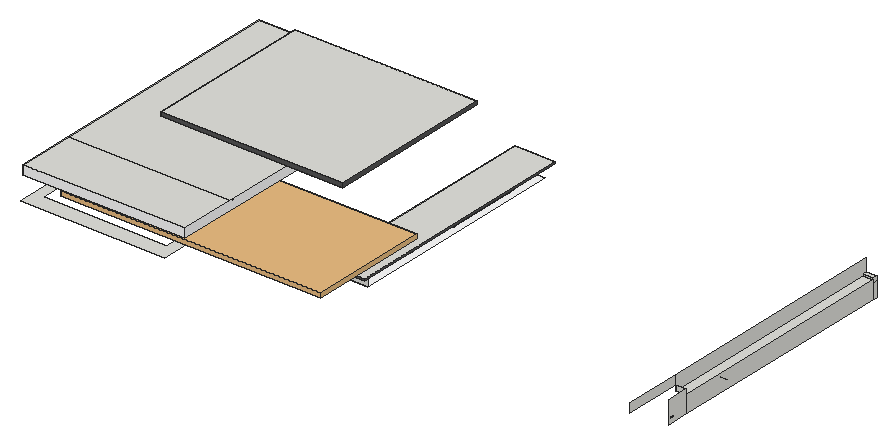
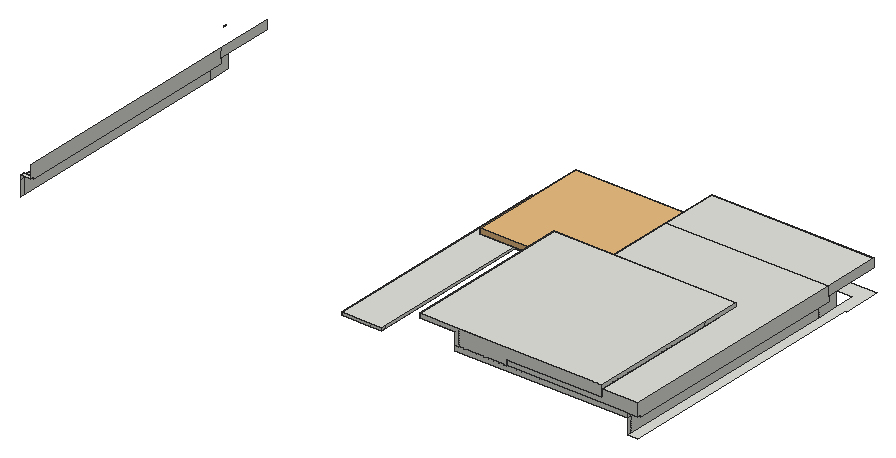
# SketchUp Ruby script. Lengths in inches.
U = 1.inch
M = Sketchup.active_model
def pt(a) = Geom::Point3d.new(a.map { |v| v * U })
def face(e, loops, mat)
  f = e.add_face(loops[0].map { |a| pt(a) })
  loops[1..].each { |l| e.add_face(l.map { |a| pt(a) }).erase! }
  f.material = f.back_material = mat if mat
  f
end
# faces: each face lists its corners as indices into pts; further lists are holes
def faces(e, pts, list, mat = nil) = list.each { |f| face(e, (f[0].is_a?(Array) ? f : [f]).map { |l| l.map { |i| pts[i] } }, mat) }
# xy, xz, yz: faces in a plane at the given z, y or x. An outline is a flat list of corners, or four numbers for a rectangle; further outlines are holes
def ring(l) = l.size == 4 ? [[l[0], l[1]], [l[2], l[1]], [l[2], l[3]], [l[0], l[3]]] : l.each_slice(2).to_a
def flat(e, list, mat, &to3) = list.each { |f| face(e, (f[0].is_a?(Array) ? f : [f]).map { |l| ring(l).map { |u, v| to3.(u, v) } }, mat) }
def xy(e, z, list, mat = nil) = flat(e, list, mat) { |x, y| [x, y, z] }
def xz(e, y, list, mat = nil) = flat(e, list, mat) { |x, z| [x, y, z] }
def yz(e, x, list, mat = nil) = flat(e, list, mat) { |y, z| [x, y, z] }
def lines(e, pts, list) = list.each { |a, b| e.add_line(pt(pts[a]), pt(pts[b])) }
# prism: a flat outline (further loops are holes) pulled along v
def prism(e, loops, v, mat = nil)
  f = face(e, loops, mat); d = Geom::Vector3d.new(v.map { |x| x * U })
  f.pushpull(f.normal.samedirection?(d) ? d.length : -d.length)
end
def box(e, o, s, mat = nil) = prism(e, [[o, [o[0] + s[0], o[1], o[2]], [o[0] + s[0], o[1] + s[1], o[2]], [o[0], o[1] + s[1], o[2]]]], [0, 0, s[2]], mat)
def at(x, y, z, deg = 0) = Geom::Transformation.translation(pt([x, y, z])) * Geom::Transformation.rotation(ORIGIN, Z_AXIS, deg.degrees)
def axes(o, x, y, z) = Geom::Transformation.new([*x, 0, *y, 0, *z, 0, *pt(o).to_a, 1])
def part(name) = M.definitions.add(name)
# library, detail: a bought-in or finely detailed component or shape, given as its bounding box
def library(name, o, s) = part(name).tap { |d| box(d.entities, o, s) }
def detail(e, o, s) = box(e.add_group.entities, o, s)
def put(e, d, t, mat = nil) = e.add_instance(d, t).tap { |i| i.material = mat if mat }
def group(e, t, mat = nil) = e.add_group.tap { |g| g.transformation = t; g.material = mat if mat }.entities
root = M.entities
M.materials.add("[Color M00]").color = [255, 255, 255]
M.materials.add("[Color M06]").color = [86, 86, 86]
c1 = library("Mesh Light\#4",[-0.5,-0.5,-0.1],[1,1,0.2])
c2 = part("Group\#24")
xy(c2.entities,0,[[203.13,95.41,201.58,95.62,200.13,96.22,198.89,97.17,197.9375,98.41,197.34,99.86,197.13,101.41,197.34,102.96,197.9375,104.41,198.89,105.65,200.13,106.61,201.58,107.21,203.13,107.41,204.6875,107.21,206.13,106.61,207.375,105.65,208.33,104.41,208.93,102.96,209.13,101.41,208.93,99.86,208.33,98.41,207.375,97.17,206.13,96.22,204.6875,95.62],[281.57,95.41,280.02,95.62,278.57,96.22,277.33,97.17,276.375,98.41,275.77,99.86,275.57,101.41,275.77,102.96,276.375,104.41,277.33,105.65,278.57,106.61,280.02,107.21,281.57,107.41,283.125,107.21,284.57,106.61,285.8125,105.65,286.77,104.41,287.37,102.96,287.57,101.41,287.37,99.86,286.77,98.41,285.8125,97.17,284.57,96.22,283.125,95.62],[350.95,95.41,349.39,95.62,347.95,96.22,346.7,97.17,345.75,98.41,345.15,99.86,344.95,101.41,345.15,102.96,345.75,104.41,346.7,105.65,347.95,106.61,349.39,107.21,350.95,107.41,352.5,107.21,353.95,106.61,355.1875,105.65,356.14,104.41,356.74,102.96,356.95,101.41,356.74,99.86,356.14,98.41,355.1875,97.17,353.95,96.22,352.5,95.62],[376,162.85,374.44,163.05,373,163.65,371.75,164.6,370.8,165.85,370.2,167.29,370,168.85,370.2,170.4,370.8,171.85,371.75,173.09,373,174.04,374.44,174.64,376,174.85,377.55,174.64,379,174.04,380.24,173.09,381.19,171.85,381.79,170.4,382,168.85,381.79,167.29,381.19,165.85,380.24,164.6,379,163.65,377.55,163.05]],"[Color M00]")
xy(c2.entities,33.4375,[[6,0,4.45,0.2,3,0.8,1.76,1.76,0.8,3,0.2,4.45,0,6,0.2,7.55,0.8,9,1.76,10.24,3,11.2,4.45,11.8,6,12,7.55,11.8,9,11.2,10.24,10.24,11.2,9,11.8,7.55,12,6,11.8,4.45,11.2,3,10.24,1.76,9,0.8,7.55,0.2],[83.125,0,81.57,0.2,80.125,0.8,78.88,1.76,77.93,3,77.33,4.45,77.125,6,77.33,7.55,77.93,9,78.88,10.24,80.125,11.2,81.57,11.8,83.125,12,84.68,11.8,86.125,11.2,87.37,10.24,88.32,9,88.92,7.55,89.125,6,88.92,4.45,88.32,3,87.37,1.76,86.125,0.8,84.68,0.2],[166.6875,0,165.13,0.2,163.6875,0.8,162.44,1.76,161.49,3,160.89,4.45,160.6875,6,160.89,7.55,161.49,9,162.44,10.24,163.6875,11.2,165.13,11.8,166.6875,12,168.24,11.8,169.6875,11.2,170.93,10.24,171.88,9,172.48,7.55,172.6875,6,172.48,4.45,171.88,3,170.93,1.76,169.6875,0.8,168.24,0.2],[166.6875,88.9375,165.13,89.14,163.6875,89.74,162.44,90.69,161.49,91.9375,160.89,93.38,160.6875,94.9375,160.89,96.49,161.49,97.9375,162.44,99.18,163.6875,100.13,165.13,100.73,166.6875,100.9375,168.24,100.73,169.6875,100.13,170.93,99.18,171.88,97.9375,172.48,96.49,172.6875,94.9375,172.48,93.38,171.88,91.9375,170.93,90.69,169.6875,89.74,168.24,89.14]],"[Color M00]")
put(c2.entities,c1,axes([191,87.42,16.72],[382.99758,0,0],[0,175.84579,0],[0,0,34.4375]))
c3 = library("Group\#23",[-0.5,-0.5,-0.1],[13,110.375,0.2])
xy(root,269.375,[[278.36,1583.41,490.8,1583.41,490.8,1676.03,484.3,1676.03,484.3,1705.53,475.29,1705.53,475.29,1606.6875,294.47,1606.6875,294.47,2020.66,279.74,2020.66,279.74,1638.35,278.36,1638.35],[484.3,1676.03,490.8,1730.6]])
xy(root,269.375,[[[490.8,1676.03,490.8,1730.6,674.49,1730.6,674.49,2001.02,715.11,2001.02,715.11,1676.03],[604.45,1698.07,606.01,1698.28,607.45,1698.875,608.7,1699.83,609.65,1701.07,610.25,1702.52,610.45,1704.07,610.25,1705.625,609.65,1707.07,608.7,1708.3125,607.45,1709.27,606.01,1709.87,604.45,1710.07,602.9,1709.87,601.45,1709.27,600.21,1708.3125,599.26,1707.07,598.66,1705.625,598.45,1704.07,598.66,1702.52,599.26,1701.07,600.21,1699.83,601.45,1698.875,602.9,1698.28],[673.83,1698.07,675.38,1698.28,676.83,1698.875,678.07,1699.83,679.02,1701.07,679.625,1702.52,679.83,1704.07,679.625,1705.625,679.02,1707.07,678.07,1708.3125,676.83,1709.27,675.38,1709.87,673.83,1710.07,672.27,1709.87,670.83,1709.27,669.59,1708.3125,668.63,1707.07,668.03,1705.625,667.83,1704.07,668.03,1702.52,668.63,1701.07,669.59,1699.83,670.83,1698.875,672.27,1698.28],[526.02,1698.07,527.57,1698.28,529.02,1698.875,530.26,1699.83,531.21,1701.07,531.8125,1702.52,532.02,1704.07,531.8125,1705.625,531.21,1707.07,530.26,1708.3125,529.02,1709.27,527.57,1709.87,526.02,1710.07,524.46,1709.87,523.02,1709.27,521.77,1708.3125,520.82,1707.07,520.22,1705.625,520.02,1704.07,520.22,1702.52,520.82,1701.07,521.77,1699.83,523.02,1698.875,524.46,1698.28],[698.88,1943.32,700.43,1943.52,701.88,1944.12,703.12,1945.08,704.08,1946.32,704.68,1947.77,704.88,1949.32,704.68,1950.87,704.08,1952.32,703.12,1953.5625,701.88,1954.51,700.43,1955.11,698.88,1955.32,697.33,1955.11,695.88,1954.51,694.64,1953.5625,693.68,1952.32,693.08,1950.87,692.88,1949.32,693.08,1947.77,693.68,1946.32,694.64,1945.08,695.88,1944.12,697.33,1943.52],[698.88,1765.51,700.43,1765.71,701.88,1766.31,703.12,1767.26,704.08,1768.51,704.68,1769.95,704.88,1771.51,704.68,1773.06,704.08,1774.51,703.12,1775.75,701.88,1776.7,700.43,1777.3,698.88,1777.51,697.33,1777.3,695.88,1776.7,694.64,1775.75,693.68,1774.51,693.08,1773.06,692.88,1771.51,693.08,1769.95,693.68,1768.51,694.64,1767.26,695.88,1766.31,697.33,1765.71],[698.88,1845.94,700.43,1846.15,701.88,1846.75,703.12,1847.7,704.08,1848.94,704.68,1850.39,704.88,1851.94,704.68,1853.5,704.08,1854.94,703.12,1856.1875,701.88,1857.14,700.43,1857.74,698.88,1857.94,697.33,1857.74,695.88,1857.14,694.64,1856.1875,693.68,1854.94,693.08,1853.5,692.88,1851.94,693.08,1850.39,693.68,1848.94,694.64,1847.7,695.88,1846.75,697.33,1846.15]]],"[Color M00]")
xy(root,279.25,[[484.3,1669.78,715.11,1676.03],[484.3,1676.03,484.3,1775.97,655.66,1775.97,655.66,2020.66,715.11,2020.66,715.11,1676.03]])
xy(root,282.6875,[[484.3,1669.78,715.11,1669.78,715.11,2020.66,655.66,2020.66,655.66,1775.97,484.3,1775.97]])
xy(root,291.125,[[304.78,1733.11,304.78,2014.29,471.68,2014.29,471.68,1853.85,462.15,1853.85,462.15,1733.11],[471.68,1853.85,542.11,2014.29]])
xy(root,294.9375,[[279.74,1669.84,294.47,2014.29],[1172.33,1669.84,1187.0625,2014.29]])
xy(root,297.875,[[279.74,2014.29,294.47,2020.66],[294.47,2014.29,471.68,2020.66],[471.68,2014.29,542.11,2020.66],[1172.33,2014.29,1187.0625,2020.66]])
xy(root,302.8125,[[[279.74,1586.53,279.74,1669.84,294.47,1669.84,294.47,1638.53,471.68,1638.53,471.68,1831.47,518.11,1831.47,518.11,1586.53],[328.88,1602.66,330.44,1602.86,331.88,1603.46,333.125,1604.42,334.08,1605.66,334.68,1607.11,334.88,1608.66,334.68,1610.21,334.08,1611.66,333.125,1612.9,331.88,1613.86,330.44,1614.46,328.88,1614.66,327.33,1614.46,325.88,1613.86,324.64,1612.9,323.6875,1611.66,323.09,1610.21,322.88,1608.66,323.09,1607.11,323.6875,1605.66,324.64,1604.42,325.88,1603.46,327.33,1602.86],[406.01,1602.66,407.56,1602.86,409.01,1603.46,410.25,1604.42,411.2,1605.66,411.8,1607.11,412.01,1608.66,411.8,1610.21,411.2,1611.66,410.25,1612.9,409.01,1613.86,407.56,1614.46,406.01,1614.66,404.45,1614.46,403.01,1613.86,401.76,1612.9,400.8125,1611.66,400.21,1610.21,400.01,1608.66,400.21,1607.11,400.8125,1605.66,401.76,1604.42,403.01,1603.46,404.45,1602.86],[489.57,1602.66,491.12,1602.86,492.57,1603.46,493.8125,1604.42,494.77,1605.66,495.37,1607.11,495.57,1608.66,495.37,1610.21,494.77,1611.66,493.8125,1612.9,492.57,1613.86,491.12,1614.46,489.57,1614.66,488.02,1614.46,486.57,1613.86,485.33,1612.9,484.375,1611.66,483.77,1610.21,483.57,1608.66,483.77,1607.11,484.375,1605.66,485.33,1604.42,486.57,1603.46,488.02,1602.86],[489.57,1691.6,491.12,1691.8,492.57,1692.4,493.8125,1693.35,494.77,1694.6,495.37,1696.04,495.57,1697.6,495.37,1699.15,494.77,1700.6,493.8125,1701.84,492.57,1702.79,491.12,1703.39,489.57,1703.6,488.02,1703.39,486.57,1702.79,485.33,1701.84,484.375,1700.6,483.77,1699.15,483.57,1697.6,483.77,1696.04,484.375,1694.6,485.33,1693.35,486.57,1692.4,488.02,1691.8]]],"[Color M00]")
xy(root,305.625,[[332.11,1831.47,471.68,2020.66]])
xy(root,316.0625,[[279.74,1586.53,518.11,1669.84],[279.74,1669.84,518.11,1669.84,518.11,1773.85,332.11,1773.85,332.11,2020.66,279.74,2020.66],[518.11,1773.85,518.11,1831.47,548.11,1831.47,548.11,2020.66,599.68,2020.66,599.68,1773.85]])
xy(root,321.8125,[[332.11,1773.85,599.68,2020.66]])
xz(root,1586.53,[[279.74,302.8125,518.11,316.0625]],"[Color M00]")
xz(root,1669.78,[[484.3,279.25,715.11,282.6875]],"[Color M06]")
xz(root,1669.84,[[279.74,294.9375,294.47,302.8125],[1172.33,294.9375,1187.0625,302.8125]])
xz(root,1676.03,[[484.3,269.375,715.11,279.25]])
xz(root,1773.85,[[332.11,316.0625,599.68,321.8125]],"[Color M06]")
xz(root,1775.97,[[484.3,279.25,655.66,282.6875]])
xz(root,1831.47,[[471.68,302.8125,518.11,305.625]])
xz(root,2014.29,[[294.47,291.125,471.68,297.875],[471.68,291.125,542.11,297.875],[279.74,294.9375,294.47,297.875],[1172.33,294.9375,1187.0625,297.875]])
xz(root,2020.66,[[655.66,279.25,671.36,282.6875],[671.36,279.25,715.11,282.6875],[294.47,291.125,548.11,297.875],[279.74,297.875,279.74,316.0625,332.11,316.0625,332.11,305.625,471.68,305.625,471.68,297.875],[471.68,297.875,471.68,305.625,332.11,305.625,332.11,321.8125,542.11,321.8125,542.11,297.875],
  [542.11,297.875,542.11,321.8125,599.68,321.8125,599.68,316.0625,548.11,316.0625,548.11,297.875]])
yz(root,279.74,[[1669.84,294.9375,1669.84,316.0625,2020.66,316.0625,2020.66,297.875,2014.29,297.875,2014.29,294.9375],[1586.53,302.8125,1669.84,316.0625]])
yz(root,294.47,[[1638.53,269.375,1669.84,302.8125],[1669.84,269.375,2014.29,294.9375],[2014.29,269.375,2020.66,291.125],[2014.29,291.125,2020.66,297.875]])
yz(root,332.11,[[1803.47,305.625,1831.47,316.0625],[1831.47,305.625,2020.66,316.0625],[1773.85,316.0625,1831.47,321.8125],[1831.47,316.0625,2020.66,321.8125]])
yz(root,471.68,[[1831.47,291.125,2014.29,297.875],[1831.47,297.875,2020.66,305.625]])
yz(root,484.3,[[1669.78,279.25,1775.97,282.6875]])
yz(root,518.11,[[1586.53,302.8125,1831.47,316.0625]],"[Color M00]")
yz(root,599.68,[[1773.85,316.0625,2020.66,321.8125]],"[Color M06]")
yz(root,655.66,[[1775.97,279.25,2014.29,282.6875],[2014.29,279.25,2020.66,282.6875]])
yz(root,715.11,[[1669.78,279.25,2020.66,282.6875]],"[Color M06]")
yz(root,1172.33,[[1669.84,294.9375,1669.84,316.0625,2020.66,316.0625,2020.66,297.875,2014.29,297.875,2014.29,294.9375],[1586.53,302.8125,1669.84,316.0625]])
yz(root,1187.0625,[[1638.53,269.375,1669.84,302.8125],[1669.84,269.375,2014.29,294.9375],[2014.29,269.375,2020.66,291.125],[2014.29,291.125,2020.66,297.875]])
p = [[526.02,1698.07,269.375],[524.46,1698.28,269.375],[524.46,1698.28,270.0625],[526.02,1698.07,270.0625],[527.57,1698.28,269.375],[527.57,1698.28,270.0625],
  [604.45,1698.07,269.375],[602.9,1698.28,269.375],[602.9,1698.28,270.0625],[604.45,1698.07,270.0625],[606.01,1698.28,269.375],[606.01,1698.28,270.0625],
  [673.83,1698.07,269.375],[672.27,1698.28,269.375],[672.27,1698.28,270.0625],[673.83,1698.07,270.0625],[675.38,1698.28,269.375],[675.38,1698.28,270.0625],
  [523.02,1698.875,269.375],[523.02,1698.875,270.0625],[529.02,1698.875,269.375],[529.02,1698.875,270.0625],[601.45,1698.875,269.375],[601.45,1698.875,270.0625],
  [607.45,1698.875,269.375],[607.45,1698.875,270.0625],[670.83,1698.875,269.375],[670.83,1698.875,270.0625],[676.83,1698.875,269.375],[676.83,1698.875,270.0625],
  [521.77,1699.83,269.375],[521.77,1699.83,270.0625],[530.26,1699.83,269.375],[530.26,1699.83,270.0625],[600.21,1699.83,269.375],[600.21,1699.83,270.0625],
  [608.7,1699.83,269.375],[608.7,1699.83,270.0625],[669.59,1699.83,269.375],[669.59,1699.83,270.0625],[678.07,1699.83,269.375],[678.07,1699.83,270.0625],
  [520.82,1701.07,269.375],[520.82,1701.07,270.0625],[531.21,1701.07,269.375],[531.21,1701.07,270.0625],[599.26,1701.07,269.375],[599.26,1701.07,270.0625],
  [609.65,1701.07,269.375],[609.65,1701.07,270.0625],[668.63,1701.07,269.375],[668.63,1701.07,270.0625],[679.02,1701.07,269.375],[679.02,1701.07,270.0625],
  [520.22,1702.52,269.375],[520.22,1702.52,270.0625],[531.8125,1702.52,269.375],[531.8125,1702.52,270.0625],[598.66,1702.52,269.375],[598.66,1702.52,270.0625],
  [610.25,1702.52,269.375],[610.25,1702.52,270.0625],[668.03,1702.52,269.375],[668.03,1702.52,270.0625],[679.625,1702.52,269.375],[679.625,1702.52,270.0625],
  [520.02,1704.07,269.375],[520.02,1704.07,270.0625],[532.02,1704.07,269.375],[532.02,1704.07,270.0625],[598.45,1704.07,269.375],[598.45,1704.07,270.0625],
  [610.45,1704.07,269.375],[610.45,1704.07,270.0625],[667.83,1704.07,269.375],[667.83,1704.07,270.0625],[679.83,1704.07,269.375],[679.83,1704.07,270.0625],
  [520.22,1705.625,269.375],[520.22,1705.625,270.0625],[531.8125,1705.625,269.375],[531.8125,1705.625,270.0625],[598.66,1705.625,269.375],[598.66,1705.625,270.0625],
  [610.25,1705.625,269.375],[610.25,1705.625,270.0625],[668.03,1705.625,269.375],[668.03,1705.625,270.0625],[679.625,1705.625,269.375],[679.625,1705.625,270.0625],
  [520.82,1707.07,269.375],[520.82,1707.07,270.0625],[531.21,1707.07,269.375],[531.21,1707.07,270.0625],[599.26,1707.07,269.375],[599.26,1707.07,270.0625],
  [609.65,1707.07,269.375],[609.65,1707.07,270.0625],[668.63,1707.07,269.375],[668.63,1707.07,270.0625],[679.02,1707.07,269.375],[679.02,1707.07,270.0625],
  [521.77,1708.3125,269.375],[521.77,1708.3125,270.0625],[530.26,1708.3125,269.375],[530.26,1708.3125,270.0625],[600.21,1708.3125,269.375],[600.21,1708.3125,270.0625],
  [608.7,1708.3125,269.375],[608.7,1708.3125,270.0625],[669.59,1708.3125,269.375],[669.59,1708.3125,270.0625],[678.07,1708.3125,269.375],[678.07,1708.3125,270.0625],
  [523.02,1709.27,269.375],[523.02,1709.27,270.0625],[529.02,1709.27,269.375],[529.02,1709.27,270.0625],[601.45,1709.27,269.375],[601.45,1709.27,270.0625],
  [607.45,1709.27,269.375],[607.45,1709.27,270.0625],[670.83,1709.27,269.375],[670.83,1709.27,270.0625],[676.83,1709.27,269.375],[676.83,1709.27,270.0625],
  [524.46,1709.87,269.375],[524.46,1709.87,270.0625],[527.57,1709.87,269.375],[527.57,1709.87,270.0625],[602.9,1709.87,269.375],[602.9,1709.87,270.0625],
  [606.01,1709.87,269.375],[606.01,1709.87,270.0625],[672.27,1709.87,269.375],[672.27,1709.87,270.0625],[675.38,1709.87,269.375],[675.38,1709.87,270.0625],
  [526.02,1710.07,269.375],[526.02,1710.07,270.0625],[604.45,1710.07,269.375],[604.45,1710.07,270.0625],[673.83,1710.07,269.375],[673.83,1710.07,270.0625],
  [698.88,1765.51,269.375],[697.33,1765.71,269.375],[697.33,1765.71,270.0625],[698.88,1765.51,270.0625],[700.43,1765.71,269.375],[700.43,1765.71,270.0625],
  [695.88,1766.31,269.375],[695.88,1766.31,270.0625],[701.88,1766.31,269.375],[701.88,1766.31,270.0625],[694.64,1767.26,269.375],[694.64,1767.26,270.0625],
  [703.12,1767.26,269.375],[703.12,1767.26,270.0625],[693.68,1768.51,269.375],[693.68,1768.51,270.0625],[704.08,1768.51,269.375],[704.08,1768.51,270.0625],
  [693.08,1769.95,269.375],[693.08,1769.95,270.0625],[704.68,1769.95,269.375],[704.68,1769.95,270.0625],[692.88,1771.51,269.375],[692.88,1771.51,270.0625],
  [704.88,1771.51,269.375],[704.88,1771.51,270.0625],[693.08,1773.06,269.375],[693.08,1773.06,270.0625],[704.68,1773.06,269.375],[704.68,1773.06,270.0625],
  [693.68,1774.51,269.375],[693.68,1774.51,270.0625],[704.08,1774.51,269.375],[704.08,1774.51,270.0625],[694.64,1775.75,269.375],[694.64,1775.75,270.0625],
  [703.12,1775.75,269.375],[703.12,1775.75,270.0625],[695.88,1776.7,269.375],[695.88,1776.7,270.0625],[701.88,1776.7,269.375],[701.88,1776.7,270.0625],
  [697.33,1777.3,269.375],[697.33,1777.3,270.0625],[700.43,1777.3,269.375],[700.43,1777.3,270.0625],[698.88,1777.51,269.375],[698.88,1777.51,270.0625],
  [698.88,1845.94,269.375],[697.33,1846.15,269.375],[697.33,1846.15,270.0625],[698.88,1845.94,270.0625],[700.43,1846.15,269.375],[700.43,1846.15,270.0625],
  [695.88,1846.75,269.375],[695.88,1846.75,270.0625],[701.88,1846.75,269.375],[701.88,1846.75,270.0625],[694.64,1847.7,269.375],[694.64,1847.7,270.0625],
  [703.12,1847.7,269.375],[703.12,1847.7,270.0625],[693.68,1848.94,269.375],[693.68,1848.94,270.0625],[704.08,1848.94,269.375],[704.08,1848.94,270.0625],
  [693.08,1850.39,269.375],[693.08,1850.39,270.0625],[704.68,1850.39,269.375],[704.68,1850.39,270.0625],[692.88,1851.94,269.375],[692.88,1851.94,270.0625],
  [704.88,1851.94,269.375],[704.88,1851.94,270.0625],[693.08,1853.5,269.375],[693.08,1853.5,270.0625],[704.68,1853.5,269.375],[704.68,1853.5,270.0625],
  [693.68,1854.94,269.375],[693.68,1854.94,270.0625],[704.08,1854.94,269.375],[704.08,1854.94,270.0625],[694.64,1856.1875,269.375],[694.64,1856.1875,270.0625],
  [703.12,1856.1875,269.375],[703.12,1856.1875,270.0625],[695.88,1857.14,269.375],[695.88,1857.14,270.0625],[701.88,1857.14,269.375],[701.88,1857.14,270.0625],
  [697.33,1857.74,269.375],[697.33,1857.74,270.0625],[700.43,1857.74,269.375],[700.43,1857.74,270.0625],[698.88,1857.94,269.375],[698.88,1857.94,270.0625],
  [698.88,1943.32,269.375],[697.33,1943.52,269.375],[697.33,1943.52,270.0625],[698.88,1943.32,270.0625],[700.43,1943.52,269.375],[700.43,1943.52,270.0625],
  [695.88,1944.12,269.375],[695.88,1944.12,270.0625],[701.88,1944.12,269.375],[701.88,1944.12,270.0625],[694.64,1945.08,269.375],[694.64,1945.08,270.0625],
  [703.12,1945.08,269.375],[703.12,1945.08,270.0625],[693.68,1946.32,269.375],[693.68,1946.32,270.0625],[704.08,1946.32,269.375],[704.08,1946.32,270.0625],
  [693.08,1947.77,269.375],[693.08,1947.77,270.0625],[704.68,1947.77,269.375],[704.68,1947.77,270.0625],[692.88,1949.32,269.375],[692.88,1949.32,270.0625],
  [704.88,1949.32,269.375],[704.88,1949.32,270.0625],[693.08,1950.87,269.375],[693.08,1950.87,270.0625],[704.68,1950.87,269.375],[704.68,1950.87,270.0625],
  [693.68,1952.32,269.375],[693.68,1952.32,270.0625],[704.08,1952.32,269.375],[704.08,1952.32,270.0625],[694.64,1953.5625,269.375],[694.64,1953.5625,270.0625],
  [703.12,1953.5625,269.375],[703.12,1953.5625,270.0625],[695.88,1954.51,269.375],[695.88,1954.51,270.0625],[701.88,1954.51,269.375],[701.88,1954.51,270.0625],
  [697.33,1955.11,269.375],[697.33,1955.11,270.0625],[700.43,1955.11,269.375],[700.43,1955.11,270.0625],[698.88,1955.32,269.375],[698.88,1955.32,270.0625],
  [328.88,1602.66,302.8125],[327.33,1602.86,302.8125],[327.33,1602.86,303.5],[328.88,1602.66,303.5],[330.44,1602.86,302.8125],[330.44,1602.86,303.5],
  [406.01,1602.66,302.8125],[404.45,1602.86,302.8125],[404.45,1602.86,303.5],[406.01,1602.66,303.5],[407.56,1602.86,302.8125],[407.56,1602.86,303.5],
  [489.57,1602.66,302.8125],[488.02,1602.86,302.8125],[488.02,1602.86,303.5],[489.57,1602.66,303.5],[491.12,1602.86,302.8125],[491.12,1602.86,303.5],
  [325.88,1603.46,302.8125],[325.88,1603.46,303.5],[331.88,1603.46,302.8125],[331.88,1603.46,303.5],[403.01,1603.46,302.8125],[403.01,1603.46,303.5],
  [409.01,1603.46,302.8125],[409.01,1603.46,303.5],[486.57,1603.46,302.8125],[486.57,1603.46,303.5],[492.57,1603.46,302.8125],[492.57,1603.46,303.5],
  [324.64,1604.42,302.8125],[324.64,1604.42,303.5],[333.125,1604.42,302.8125],[333.125,1604.42,303.5],[401.76,1604.42,302.8125],[401.76,1604.42,303.5],
  [410.25,1604.42,302.8125],[410.25,1604.42,303.5],[485.33,1604.42,302.8125],[485.33,1604.42,303.5],[493.8125,1604.42,302.8125],[493.8125,1604.42,303.5],
  [323.6875,1605.66,302.8125],[323.6875,1605.66,303.5],[334.08,1605.66,302.8125],[334.08,1605.66,303.5],[400.8125,1605.66,302.8125],[400.8125,1605.66,303.5],
  [411.2,1605.66,302.8125],[411.2,1605.66,303.5],[484.375,1605.66,302.8125],[484.375,1605.66,303.5],[494.77,1605.66,302.8125],[494.77,1605.66,303.5],
  [323.09,1607.11,302.8125],[323.09,1607.11,303.5],[334.68,1607.11,302.8125],[334.68,1607.11,303.5],[400.21,1607.11,302.8125],[400.21,1607.11,303.5],
  [411.8,1607.11,302.8125],[411.8,1607.11,303.5],[483.77,1607.11,302.8125],[483.77,1607.11,303.5],[495.37,1607.11,302.8125],[495.37,1607.11,303.5],
  [322.88,1608.66,302.8125],[322.88,1608.66,303.5],[334.88,1608.66,302.8125],[334.88,1608.66,303.5],[400.01,1608.66,302.8125],[400.01,1608.66,303.5],
  [412.01,1608.66,302.8125],[412.01,1608.66,303.5],[483.57,1608.66,302.8125],[483.57,1608.66,303.5],[495.57,1608.66,302.8125],[495.57,1608.66,303.5],
  [1215.68,1607.11,302.8125],[1215.47,1608.66,302.8125],[1215.47,1608.66,303.5],[1215.68,1607.11,303.5],[323.09,1610.21,302.8125],[323.09,1610.21,303.5],
  [334.68,1610.21,302.8125],[334.68,1610.21,303.5],[400.21,1610.21,302.8125],[400.21,1610.21,303.5],[411.8,1610.21,302.8125],[411.8,1610.21,303.5],
  [483.77,1610.21,302.8125],[483.77,1610.21,303.5],[495.37,1610.21,302.8125],[495.37,1610.21,303.5],[1215.68,1610.21,302.8125],[1215.68,1610.21,303.5],
  [323.6875,1611.66,302.8125],[323.6875,1611.66,303.5],[334.08,1611.66,302.8125],[334.08,1611.66,303.5],[400.8125,1611.66,302.8125],[400.8125,1611.66,303.5],
  [411.2,1611.66,302.8125],[411.2,1611.66,303.5],[484.375,1611.66,302.8125],[484.375,1611.66,303.5],[494.77,1611.66,302.8125],[494.77,1611.66,303.5],
  [324.64,1612.9,302.8125],[324.64,1612.9,303.5],[333.125,1612.9,302.8125],[333.125,1612.9,303.5],[401.76,1612.9,302.8125],[401.76,1612.9,303.5],
  [410.25,1612.9,302.8125],[410.25,1612.9,303.5],[485.33,1612.9,302.8125],[485.33,1612.9,303.5],[493.8125,1612.9,302.8125],[493.8125,1612.9,303.5],
  [325.88,1613.86,302.8125],[325.88,1613.86,303.5],[331.88,1613.86,302.8125],[331.88,1613.86,303.5],[403.01,1613.86,302.8125],[403.01,1613.86,303.5],
  [409.01,1613.86,302.8125],[409.01,1613.86,303.5],[486.57,1613.86,302.8125],[486.57,1613.86,303.5],[492.57,1613.86,302.8125],[492.57,1613.86,303.5],
  [327.33,1614.46,302.8125],[327.33,1614.46,303.5],[330.44,1614.46,302.8125],[330.44,1614.46,303.5],[404.45,1614.46,302.8125],[404.45,1614.46,303.5],
  [407.56,1614.46,302.8125],[407.56,1614.46,303.5],[488.02,1614.46,302.8125],[488.02,1614.46,303.5],[491.12,1614.46,302.8125],[491.12,1614.46,303.5],
  [328.88,1614.66,302.8125],[328.88,1614.66,303.5],[406.01,1614.66,302.8125],[406.01,1614.66,303.5],[489.57,1614.66,302.8125],[489.57,1614.66,303.5],
  [489.57,1691.6,302.8125],[488.02,1691.8,302.8125],[488.02,1691.8,303.5],[489.57,1691.6,303.5],[491.12,1691.8,302.8125],[491.12,1691.8,303.5],
  [486.57,1692.4,302.8125],[486.57,1692.4,303.5],[492.57,1692.4,302.8125],[492.57,1692.4,303.5],[485.33,1693.35,302.8125],[485.33,1693.35,303.5],
  [493.8125,1693.35,302.8125],[493.8125,1693.35,303.5],[484.375,1694.6,302.8125],[484.375,1694.6,303.5],[494.77,1694.6,302.8125],[494.77,1694.6,303.5],
  [483.77,1696.04,302.8125],[483.77,1696.04,303.5],[495.37,1696.04,302.8125],[495.37,1696.04,303.5],[483.57,1697.6,302.8125],[483.57,1697.6,303.5],
  [495.57,1697.6,302.8125],[495.57,1697.6,303.5],[483.77,1699.15,302.8125],[483.77,1699.15,303.5],[495.37,1699.15,302.8125],[495.37,1699.15,303.5],
  [484.375,1700.6,302.8125],[484.375,1700.6,303.5],[494.77,1700.6,302.8125],[494.77,1700.6,303.5],[485.33,1701.84,302.8125],[485.33,1701.84,303.5],
  [493.8125,1701.84,302.8125],[493.8125,1701.84,303.5],[486.57,1702.79,302.8125],[486.57,1702.79,303.5],[492.57,1702.79,302.8125],[492.57,1702.79,303.5],
  [488.02,1703.39,302.8125],[488.02,1703.39,303.5],[491.12,1703.39,302.8125],[491.12,1703.39,303.5],[489.57,1703.6,302.8125],[489.57,1703.6,303.5],
  [332.11,1803.47,305.625],[501.74,1803.47,305.625],[542.11,2014.29,297.875],[542.11,1831.47,297.875],[542.11,1853.85,291.125],[548.11,1853.85,291.125],
  [674.49,2001.02,269.375],[674.49,2001.02,277.5],[542.11,1831.47,291.125],[304.78,1733.11,291.125],[294.47,1733.11,291.125],[1197.375,1733.11,291.125],
  [1187.0625,1733.11,291.125]]
faces(root,p,[[0,1,2,3],[4,0,3,5],[6,7,8,9],[10,6,9,11],[12,13,14,15],[16,12,15,17],[1,18,19,2],[20,4,5,21],
  [7,22,23,8],[24,10,11,25],[13,26,27,14],[28,16,17,29],[18,30,31,19],[32,20,21,33],[22,34,35,23],[36,24,25,37],
  [26,38,39,27],[40,28,29,41],[30,42,43,31],[44,32,33,45],[34,46,47,35],[48,36,37,49],[38,50,51,39],[52,40,41,53],
  [42,54,55,43],[56,44,45,57],[46,58,59,47],[60,48,49,61],[50,62,63,51],[64,52,53,65],[54,66,67,55],[68,56,57,69],
  [58,70,71,59],[72,60,61,73],[62,74,75,63],[76,64,65,77],[66,78,79,67],[80,68,69,81],[70,82,83,71],[84,72,73,85],
  [74,86,87,75],[88,76,77,89],[78,90,91,79],[92,80,81,93],[82,94,95,83],[96,84,85,97],[86,98,99,87],[100,88,89,101],
  [90,102,103,91],[104,92,93,105],[94,106,107,95],[108,96,97,109],[98,110,111,99],[112,100,101,113],[102,114,115,103],[116,104,105,117],
  [106,118,119,107],[120,108,109,121],[110,122,123,111],[124,112,113,125],[114,126,127,115],[128,116,117,129],[118,130,131,119],[132,120,121,133],
  [122,134,135,123],[136,124,125,137],[126,138,139,127],[138,128,129,139],[130,140,141,131],[140,132,133,141],[134,142,143,135],[142,136,137,143],
  [144,145,146,147],[148,144,147,149],[145,150,151,146],[152,148,149,153],[150,154,155,151],[156,152,153,157],[154,158,159,155],[160,156,157,161],
  [158,162,163,159],[164,160,161,165],[162,166,167,163],[168,164,165,169],[166,170,171,167],[172,168,169,173],[170,174,175,171],[176,172,173,177],
  [174,178,179,175],[180,176,177,181],[178,182,183,179],[184,180,181,185],[182,186,187,183],[188,184,185,189],[186,190,191,187],[190,188,189,191],
  [192,193,194,195],[196,192,195,197],[193,198,199,194],[200,196,197,201],[198,202,203,199],[204,200,201,205],[202,206,207,203],[208,204,205,209],
  [206,210,211,207],[212,208,209,213],[210,214,215,211],[216,212,213,217],[214,218,219,215],[220,216,217,221],[218,222,223,219],[224,220,221,225],
  [222,226,227,223],[228,224,225,229],[226,230,231,227],[232,228,229,233],[230,234,235,231],[236,232,233,237],[234,238,239,235],[238,236,237,239],
  [240,241,242,243],[244,240,243,245],[241,246,247,242],[248,244,245,249],[246,250,251,247],[252,248,249,253],[250,254,255,251],[256,252,253,257],
  [254,258,259,255],[260,256,257,261],[258,262,263,259],[264,260,261,265],[262,266,267,263],[268,264,265,269],[266,270,271,267],[272,268,269,273],
  [270,274,275,271],[276,272,273,277],[274,278,279,275],[280,276,277,281],[278,282,283,279],[284,280,281,285],[282,286,287,283],[286,284,285,287],
  [288,289,290,291],[292,288,291,293],[294,295,296,297],[298,294,297,299],[300,301,302,303],[304,300,303,305],[289,306,307,290],[308,292,293,309],
  [295,310,311,296],[312,298,299,313],[301,314,315,302],[316,304,305,317],[306,318,319,307],[320,308,309,321],[310,322,323,311],[324,312,313,325],
  [314,326,327,315],[328,316,317,329],[318,330,331,319],[332,320,321,333],[322,334,335,323],[336,324,325,337],[326,338,339,327],[340,328,329,341],
  [330,342,343,331],[344,332,333,345],[334,346,347,335],[348,336,337,349],[338,350,351,339],[352,340,341,353],[342,354,355,343],[356,344,345,357],
  [346,358,359,347],[360,348,349,361],[350,362,363,351],[364,352,353,365],[366,367,368,369],[354,370,371,355],[372,356,357,373],[358,374,375,359],
  [376,360,361,377],[362,378,379,363],[380,364,365,381],[367,382,383,368],[370,384,385,371],[386,372,373,387],[374,388,389,375],[390,376,377,391],
  [378,392,393,379],[394,380,381,395],[384,396,397,385],[398,386,387,399],[388,400,401,389],[402,390,391,403],[392,404,405,393],[406,394,395,407],
  [396,408,409,397],[410,398,399,411],[400,412,413,401],[414,402,403,415],[404,416,417,405],[418,406,407,419],[408,420,421,409],[422,410,411,423],
  [412,424,425,413],[426,414,415,427],[416,428,429,417],[430,418,419,431],[420,432,433,421],[432,422,423,433],[424,434,435,425],[434,426,427,435],
  [428,436,437,429],[436,430,431,437],[438,439,440,441],[442,438,441,443],[439,444,445,440],[446,442,443,447],[444,448,449,445],[450,446,447,451],
  [448,452,453,449],[454,450,451,455],[452,456,457,453],[458,454,455,459],[456,460,461,457],[462,458,459,463],[460,464,465,461],[466,462,463,467],
  [464,468,469,465],[470,466,467,471],[468,472,473,469],[474,470,471,475],[472,476,477,473],[478,474,475,479],[476,480,481,477],[482,478,479,483],
  [480,484,485,481],[484,482,483,485]],"[Color M00]")
lines(root,p,[[486,487],[488,489],[490,491],[492,493],[490,494],[495,496],[497,498]])
put(root,c2,at(322.88,1602.66,270.0625))
put(root,c3,at(692.88,1845.94,270.0625))
